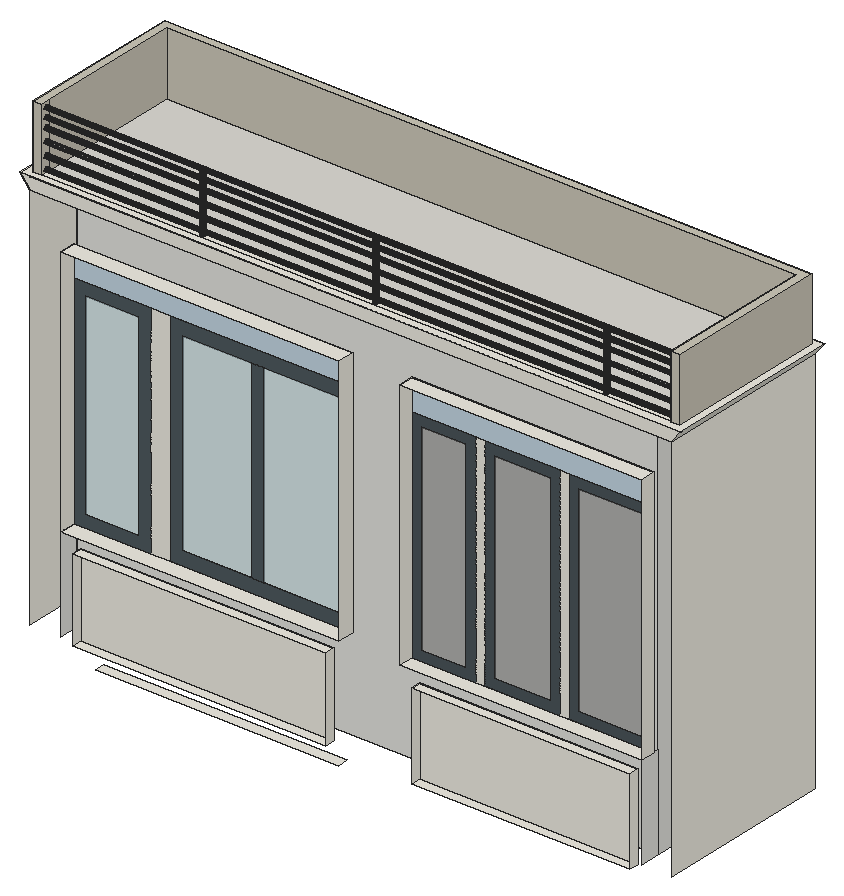
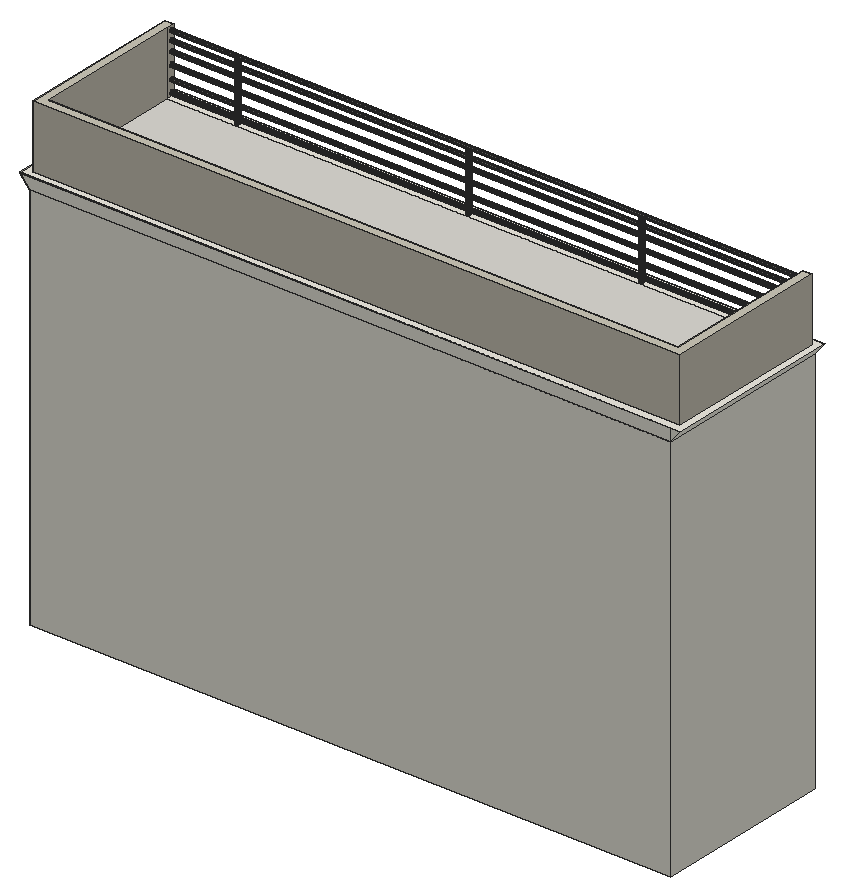
# SketchUp Ruby script. Lengths in inches.
U = 1.inch
M = Sketchup.active_model
def pt(a) = Geom::Point3d.new(a.map { |v| v * U })
def face(e, loops, mat)
  f = e.add_face(loops[0].map { |a| pt(a) })
  loops[1..].each { |l| e.add_face(l.map { |a| pt(a) }).erase! }
  f.material = f.back_material = mat if mat
  f
end
# faces: each face lists its corners as indices into pts; further lists are holes
def faces(e, pts, list, mat = nil) = list.each { |f| face(e, (f[0].is_a?(Array) ? f : [f]).map { |l| l.map { |i| pts[i] } }, mat) }
# xy, xz, yz: faces in a plane at the given z, y or x. An outline is a flat list of corners, or four numbers for a rectangle; further outlines are holes
def ring(l) = l.size == 4 ? [[l[0], l[1]], [l[2], l[1]], [l[2], l[3]], [l[0], l[3]]] : l.each_slice(2).to_a
def flat(e, list, mat, &to3) = list.each { |f| face(e, (f[0].is_a?(Array) ? f : [f]).map { |l| ring(l).map { |u, v| to3.(u, v) } }, mat) }
def xy(e, z, list, mat = nil) = flat(e, list, mat) { |x, y| [x, y, z] }
def xz(e, y, list, mat = nil) = flat(e, list, mat) { |x, z| [x, y, z] }
def yz(e, x, list, mat = nil) = flat(e, list, mat) { |y, z| [x, y, z] }
def lines(e, pts, list) = list.each { |a, b| e.add_line(pt(pts[a]), pt(pts[b])) }
# prism: a flat outline (further loops are holes) pulled along v
def prism(e, loops, v, mat = nil)
  f = face(e, loops, mat); d = Geom::Vector3d.new(v.map { |x| x * U })
  f.pushpull(f.normal.samedirection?(d) ? d.length : -d.length)
end
def box(e, o, s, mat = nil) = prism(e, [[o, [o[0] + s[0], o[1], o[2]], [o[0] + s[0], o[1] + s[1], o[2]], [o[0], o[1] + s[1], o[2]]]], [0, 0, s[2]], mat)
def at(x, y, z, deg = 0) = Geom::Transformation.translation(pt([x, y, z])) * Geom::Transformation.rotation(ORIGIN, Z_AXIS, deg.degrees)
def axes(o, x, y, z) = Geom::Transformation.new([*x, 0, *y, 0, *z, 0, *pt(o).to_a, 1])
def part(name) = M.definitions.add(name)
# library, detail: a bought-in or finely detailed component or shape, given as its bounding box
def library(name, o, s) = part(name).tap { |d| box(d.entities, o, s) }
def detail(e, o, s) = box(e.add_group.entities, o, s)
def put(e, d, t, mat = nil) = e.add_instance(d, t).tap { |i| i.material = mat if mat }
def group(e, t, mat = nil) = e.add_group.tap { |g| g.transformation = t; g.material = mat if mat }.entities
root = M.entities
M.materials.add("[Formica Graystone]").color = [204, 199, 184]
M.materials.add("[Formica Speckled Grey]1").color = [75, 84, 89]
M.materials.add("[Formica Speckled Grey]2").color = [79, 89, 94]
M.materials.add("[Granite Light Gray]").color = [149, 148, 144]
M.materials.add("[Terrazzo Light Blue]").color = [196, 214, 227]
M.materials.add("[Terrazzo Tile Light]").color = [219, 217, 210]
M.materials.add("[Tile Limestone Large]").color = [237, 234, 224]
M.materials.add("[Translucent Glass Gray]").color = [128, 128, 128]
M.materials["[Translucent Glass Gray]"].alpha = 0.5
M.materials.add("[Translucent Glass Safety]").color = [204, 235, 244]
M.materials["[Translucent Glass Safety]"].alpha = 0.5
xy(root,328.93,[[111.93,233.86,355.29,244.48]],"[Tile Limestone Large]")
xy(root,338.4,[[428.87,233.86,647.75,243.17]],"[Tile Limestone Large]")
xy(root,342.19,[[88.43,233.86,342.93,244.04]],"[Tile Limestone Large]")
xy(root,346.625,[[76.4,254.16,659.08,383.27]])
xy(root,424.46,[[428.87,233.86,647.75,243.17]],"[Tile Limestone Large]")
xy(root,425.32,[[88.43,233.86,342.93,244.04]],"[Tile Limestone Large]")
xy(root,440.5625,[[76.4,233.86,355.29,251.23],[416.36,233.86,659.08,249.23]],"[Tile Limestone Large]")
xy(root,692.2,[[76.4,233.86,355.29,251.23],[416.36,233.86,659.08,249.23]],"[Tile Limestone Large]")
xy(root,737,[[46.1875,233.86,46.1875,413.49,689.3,413.49,689.3,233.86,659.08,233.86,659.08,383.27,76.4,383.27,76.4,233.86],[76.4,233.86,659.08,254.16],[76.4,254.16,659.08,383.27],[76.4,254.16,659.08,383.27]])
xy(root,749.625,[[43.22,241.02,43.22,406.33,691.7,406.33,691.7,241.02,682.63,241.02,682.63,397.26,52.29,397.26,52.29,241.02],[209.95,243.3,209.34,243.38,208.76,243.62,208.27,244,207.9,244.49,207.66,245.0625,207.58,245.68,207.66,246.29,207.9,246.87,208.27,247.36,208.76,247.73,209.34,247.97,209.95,248.05,210.57,247.97,211.14,247.73,211.63,247.36,212.01,246.87,212.25,246.29,212.33,245.68,212.25,245.0625,212.01,244.49,211.63,244,211.14,243.62,210.57,243.38],[383.14,243.3,382.52,243.38,381.95,243.62,381.46,244,381.08,244.49,380.85,245.0625,380.76,245.68,380.85,246.29,381.08,246.87,381.46,247.36,381.95,247.73,382.52,247.97,383.14,248.05,383.75,247.97,384.33,247.73,384.82,247.36,385.2,246.87,385.43,246.29,385.51,245.68,385.43,245.0625,385.2,244.49,384.82,244,384.33,243.62,383.75,243.38],[614.64,243.3,614.02,243.38,613.45,243.62,612.96,244,612.58,244.49,612.35,245.0625,612.26,245.68,612.35,246.29,612.58,246.87,612.96,247.36,613.45,247.73,614.02,247.97,614.64,248.05,615.25,247.97,615.83,247.73,616.32,247.36,616.7,246.87,616.93,246.29,617.01,245.68,616.93,245.0625,616.7,244.49,616.32,244,615.83,243.62,615.25,243.38]])
xy(root,749.625,[[52.29,250.09,682.63,397.26]],"[Terrazzo Tile Light]")
xy(root,749.625,[[[36.0625,233.86,698.86,413.49],[43.22,241.02,691.7,406.33]],[[52.29,241.02,682.63,250.09],[614.64,243.3,614.02,243.38,613.45,243.62,612.96,244,612.58,244.49,612.35,245.0625,612.26,245.68,612.35,246.29,612.58,246.87,612.96,247.36,613.45,247.73,614.02,247.97,614.64,248.05,615.25,247.97,615.83,247.73,616.32,247.36,616.7,246.87,616.93,246.29,617.01,245.68,616.93,245.0625,616.7,244.49,616.32,244,615.83,243.62,615.25,243.38],[209.95,243.3,209.34,243.38,208.76,243.62,208.27,244,207.9,244.49,207.66,245.0625,207.58,245.68,207.66,246.29,207.9,246.87,208.27,247.36,208.76,247.73,209.34,247.97,209.95,248.05,210.57,247.97,211.14,247.73,211.63,247.36,212.01,246.87,212.25,246.29,212.33,245.68,212.25,245.0625,212.01,244.49,211.63,244,211.14,243.62,210.57,243.38],[383.14,243.3,382.52,243.38,381.95,243.62,381.46,244,381.08,244.49,380.85,245.0625,380.76,245.68,380.85,246.29,381.08,246.87,381.46,247.36,381.95,247.73,382.52,247.97,383.14,248.05,383.75,247.97,384.33,247.73,384.82,247.36,385.2,246.87,385.43,246.29,385.51,245.68,385.43,245.0625,385.2,244.49,384.82,244,384.33,243.62,383.75,243.38]]],"[Tile Limestone Large]")
xy(root,808.62,[[383.14,243.3,383.75,243.38,383.8,243.4,382.48,243.4,382.52,243.38],[382.48,243.4,383.8,243.4,384.33,243.62,384.82,244,385.2,244.49,385.43,245.0625,385.51,245.68,385.43,246.29,385.2,246.87,385.17,246.9,381.11,246.9,381.08,246.87,380.85,246.29,380.76,245.68,380.85,245.0625,381.08,244.49,381.46,244,381.95,243.62],[381.11,246.9,385.17,246.9,384.82,247.36,384.33,247.73,383.75,247.97,383.14,248.05,382.52,247.97,381.95,247.73,381.46,247.36]])
xy(root,809.09,[[209.95,243.3,210.23,243.34,209.67,243.34],[209.67,243.34,210.23,243.34,210.57,243.38,211.14,243.62,211.63,244,212.01,244.49,212.25,245.0625,212.33,245.68,212.25,246.29,212.01,246.87,211.93,246.97,207.97,246.97,207.9,246.87,207.66,246.29,207.58,245.68,207.66,245.0625,207.9,244.49,208.27,244,208.76,243.62,209.34,243.38],[207.97,246.97,211.93,246.97,211.63,247.36,211.14,247.73,210.57,247.97,209.95,248.05,209.34,247.97,208.76,247.73,208.27,247.36]])
xy(root,809.3125,[[614.64,243.3,615.25,243.38,615.83,243.62,616.32,244,616.7,244.49,616.93,245.0625,617.01,245.68,616.93,246.29,616.7,246.87,616.32,247.36,615.83,247.73,615.25,247.97,614.64,248.05,614.02,247.97,613.45,247.73,612.96,247.36,612.58,246.87,612.35,246.29,612.26,245.68,612.35,245.0625,612.58,244.49,612.96,244,613.45,243.62,614.02,243.38]])
xy(root,812.8125,[[43.22,241.02,52.29,241.02,52.29,397.26,682.63,397.26,682.63,241.02,691.7,241.02,691.7,406.33,43.22,406.33]],"[Formica Graystone]")
xz(root,233.86,[[46.1875,749.1875,698.86,749.625]])
xz(root,233.86,[[46.1875,737,689.3,737,698.86,749.1875,46.1875,749.1875,46.1875,749.625,36.0625,749.625]],"[Tile Limestone Large]")
xz(root,241.02,[[43.22,749.625,52.29,812.8125],[682.63,749.625,691.7,812.8125]],"[Formica Graystone]")
xz(root,243.17,[[428.87,338.4,647.75,424.46]],"[Tile Limestone Large]")
xz(root,244.04,[[88.43,342.19,342.93,425.32]],"[Tile Limestone Large]")
xz(root,249.23,[[[416.36,440.5625,480.46,661.07],[426.18,450.39,470.64,651.24]],[[489.4,440.5625,565.3,661.07],[499.22,450.39,555.48,651.24]],[[574.24,440.5625,659.08,661.07],[584.07,450.39,649.26,651.24]]],"[Formica Speckled Grey]1")
xz(root,249.23,[[416.36,661.07,659.08,692.2]],"[Terrazzo Light Blue]")
xz(root,249.23,[[480.46,440.5625,489.4,661.07],[565.3,440.5625,574.24,661.07]],"[Tile Limestone Large]")
xz(root,249.23,[[426.18,450.39,470.64,651.24],[499.22,450.39,555.48,651.24],[584.07,450.39,649.26,651.24]],"[Translucent Glass Gray]")
xz(root,251.23,[[[76.4,440.5625,153.38,661.07],[88.41,452.58,141.37,649.05]],[[172.06,440.5625,355.29,661.07],[185.5,454,341.85,647.625]],[254.47,454,266.69,647.625]],"[Formica Speckled Grey]2")
xz(root,251.23,[[76.4,661.07,355.29,692.2]],"[Terrazzo Light Blue]")
xz(root,251.23,[[153.38,440.5625,172.06,661.07]],"[Tile Limestone Large]")
xz(root,251.23,[[88.41,452.58,141.37,649.05],[185.5,454,254.47,647.625],[266.69,454,341.85,647.625]],"[Translucent Glass Safety]")
xz(root,254.16,[[76.4,346.625,659.08,737]])
xz(root,383.27,[[76.4,346.625,659.08,737]])
xz(root,397.26,[[52.29,749.625,682.63,812.8125]],"[Formica Graystone]")
xz(root,406.33,[[43.22,749.625,691.7,812.8125]],"[Formica Graystone]")
xz(root,413.49,[[46.1875,346.625,689.3,737],[46.1875,737,36.0625,749.625,698.86,749.625,698.86,749.1875,46.1875,749.1875],[46.1875,737,46.1875,749.1875,698.86,749.1875,689.3,737]],"[Tile Limestone Large]")
yz(root,43.22,[[241.02,749.625,406.33,812.8125]],"[Formica Graystone]")
yz(root,46.1875,[[233.86,346.625,413.49,737]],"[Tile Limestone Large]")
yz(root,52.29,[[245.15,751.4,244.68,751.46,244.25,751.65,243.87,751.93,243.58,752.31,243.4,752.75,243.34,753.22,243.4,753.68,243.58,754.12,243.87,754.5,244.25,754.78,244.68,754.97,245.15,755.03,245.62,754.97,246.06,754.78,246.43,754.5,246.72,754.12,246.9,753.68,246.97,753.22,246.9,752.75,246.72,752.31,246.43,751.93,246.06,751.65,245.62,751.46],[245.15,763.65,244.68,763.71,244.25,763.9,243.87,764.18,243.58,764.56,243.4,765,243.34,765.47,243.4,765.93,243.58,766.37,243.87,766.75,244.25,767.03,244.68,767.22,245.15,767.28,245.62,767.22,246.06,767.03,246.43,766.75,246.72,766.37,246.9,765.93,246.97,765.47,246.9,765,246.72,764.56,246.43,764.18,246.06,763.9,245.62,763.71],[245.15,776.34,244.68,776.4,244.25,776.58,243.87,776.87,243.58,777.25,243.4,777.68,243.34,778.15,243.4,778.62,243.58,779.06,243.87,779.43,244.25,779.72,244.68,779.9,245.15,779.97,245.62,779.9,246.06,779.72,246.43,779.43,246.72,779.06,246.9,778.62,246.97,778.15,246.9,777.68,246.72,777.25,246.43,776.87,246.06,776.58,245.62,776.4],[245.15,788.72,244.68,788.78,244.25,788.96,243.87,789.25,243.58,789.62,243.4,790.06,243.34,790.53,243.4,791,243.58,791.43,243.87,791.81,244.25,792.1,244.68,792.28,245.15,792.34,245.62,792.28,246.06,792.1,246.43,791.81,246.72,791.43,246.9,791,246.97,790.53,246.9,790.06,246.72,789.62,246.43,789.25,246.06,788.96,245.62,788.78],[245.15,798.28,244.68,798.34,244.25,798.52,243.87,798.81,243.58,799.18,243.4,799.62,243.34,800.09,243.4,800.56,243.58,801,243.87,801.37,244.25,801.66,244.68,801.84,245.15,801.9,245.62,801.84,246.06,801.66,246.43,801.37,246.72,801,246.9,800.56,246.97,800.09,246.9,799.62,246.72,799.18,246.43,798.81,246.06,798.52,245.62,798.34],
  [245.15,807.28,244.68,807.34,244.25,807.52,243.87,807.81,243.58,808.18,243.4,808.62,243.34,809.09,243.4,809.56,243.58,810,243.87,810.37,244.25,810.66,244.68,810.84,245.15,810.9,245.62,810.84,246.06,810.66,246.43,810.37,246.72,810,246.9,809.56,246.97,809.09,246.9,808.62,246.72,808.18,246.43,807.81,246.06,807.52,245.62,807.34]])
yz(root,52.29,[[[241.02,749.625,250.09,812.8125],[245.15,807.28,244.68,807.34,244.25,807.52,243.87,807.81,243.58,808.18,243.4,808.62,243.34,809.09,243.4,809.56,243.58,810,243.87,810.37,244.25,810.66,244.68,810.84,245.15,810.9,245.62,810.84,246.06,810.66,246.43,810.37,246.72,810,246.9,809.56,246.97,809.09,246.9,808.62,246.72,808.18,246.43,807.81,246.06,807.52,245.62,807.34],[245.15,751.4,244.68,751.46,244.25,751.65,243.87,751.93,243.58,752.31,243.4,752.75,243.34,753.22,243.4,753.68,243.58,754.12,243.87,754.5,244.25,754.78,244.68,754.97,245.15,755.03,245.62,754.97,246.06,754.78,246.43,754.5,246.72,754.12,246.9,753.68,246.97,753.22,246.9,752.75,246.72,752.31,246.43,751.93,246.06,751.65,245.62,751.46],[245.15,798.28,244.68,798.34,244.25,798.52,243.87,798.81,243.58,799.18,243.4,799.62,243.34,800.09,243.4,800.56,243.58,801,243.87,801.37,244.25,801.66,244.68,801.84,245.15,801.9,245.62,801.84,246.06,801.66,246.43,801.37,246.72,801,246.9,800.56,246.97,800.09,246.9,799.62,246.72,799.18,246.43,798.81,246.06,798.52,245.62,798.34],[245.15,763.65,244.68,763.71,244.25,763.9,243.87,764.18,243.58,764.56,243.4,765,243.34,765.47,243.4,765.93,243.58,766.37,243.87,766.75,244.25,767.03,244.68,767.22,245.15,767.28,245.62,767.22,246.06,767.03,246.43,766.75,246.72,766.37,246.9,765.93,246.97,765.47,246.9,765,246.72,764.56,246.43,764.18,246.06,763.9,245.62,763.71],[245.15,788.72,244.68,788.78,244.25,788.96,243.87,789.25,243.58,789.62,243.4,790.06,243.34,790.53,243.4,791,243.58,791.43,243.87,791.81,244.25,792.1,244.68,792.28,245.15,792.34,245.62,792.28,246.06,792.1,246.43,791.81,246.72,791.43,246.9,791,246.97,790.53,246.9,790.06,246.72,789.62,246.43,789.25,246.06,788.96,245.62,788.78],[245.15,776.34,244.68,776.4,244.25,776.58,243.87,776.87,243.58,777.25,243.4,777.68,243.34,778.15,243.4,778.62,243.58,779.06,243.87,779.43,244.25,779.72,244.68,779.9,245.15,779.97,245.62,779.9,246.06,779.72,246.43,779.43,246.72,779.06,246.9,778.62,246.97,778.15,246.9,777.68,246.72,777.25,246.43,776.87,246.06,776.58,245.62,776.4]],[250.09,749.625,397.26,812.8125]],"[Formica Graystone]")
yz(root,76.4,[[233.86,346.625,254.16,440.5625],[254.16,346.625,383.27,737]])
yz(root,76.4,[[233.86,440.5625,251.23,692.2]],"[Tile Limestone Large]")
yz(root,88.43,[[233.86,342.19,244.04,425.32]],"[Tile Limestone Large]")
yz(root,342.93,[[233.86,342.19,244.04,425.32]],"[Tile Limestone Large]")
yz(root,355.29,[[233.86,440.5625,251.23,692.2]],"[Tile Limestone Large]")
yz(root,416.36,[[233.86,440.5625,249.23,692.2]],"[Tile Limestone Large]")
yz(root,428.87,[[233.86,338.4,243.17,424.46]],"[Tile Limestone Large]")
yz(root,647.75,[[233.86,338.4,243.17,424.46]],"[Tile Limestone Large]")
yz(root,659.08,[[233.86,346.625,254.16,440.5625],[254.16,346.625,383.27,737]])
yz(root,659.08,[[233.86,440.5625,249.23,692.2]],"[Tile Limestone Large]")
yz(root,682.63,[[[241.02,749.625,250.09,812.8125],[245.15,807.28,245.62,807.34,246.06,807.52,246.43,807.81,246.72,808.18,246.9,808.62,246.97,809.09,246.9,809.56,246.72,810,246.43,810.37,246.06,810.66,245.62,810.84,245.15,810.9,244.68,810.84,244.25,810.66,243.87,810.37,243.58,810,243.4,809.56,243.34,809.09,243.4,808.62,243.58,808.18,243.87,807.81,244.25,807.52,244.68,807.34],[245.15,798.28,245.62,798.34,246.06,798.52,246.43,798.81,246.72,799.18,246.9,799.62,246.97,800.09,246.9,800.56,246.72,801,246.43,801.37,246.06,801.66,245.62,801.84,245.15,801.9,244.68,801.84,244.25,801.66,243.87,801.37,243.58,801,243.4,800.56,243.34,800.09,243.4,799.62,243.58,799.18,243.87,798.81,244.25,798.52,244.68,798.34],[245.15,788.72,245.62,788.78,246.06,788.96,246.43,789.25,246.72,789.62,246.9,790.06,246.97,790.53,246.9,791,246.72,791.43,246.43,791.81,246.06,792.1,245.62,792.28,245.15,792.34,244.68,792.28,244.25,792.1,243.87,791.81,243.58,791.43,243.4,791,243.34,790.53,243.4,790.06,243.58,789.62,243.87,789.25,244.25,788.96,244.68,788.78],[245.15,776.34,245.62,776.4,246.06,776.58,246.43,776.87,246.72,777.25,246.9,777.68,246.97,778.15,246.9,778.62,246.72,779.06,246.43,779.43,246.06,779.72,245.62,779.9,245.15,779.97,244.68,779.9,244.25,779.72,243.87,779.43,243.58,779.06,243.4,778.62,243.34,778.15,243.4,777.68,243.58,777.25,243.87,776.87,244.25,776.58,244.68,776.4],[245.15,751.4,245.62,751.46,246.06,751.65,246.43,751.93,246.72,752.31,246.9,752.75,246.97,753.22,246.9,753.68,246.72,754.12,246.43,754.5,246.06,754.78,245.62,754.97,245.15,755.03,244.68,754.97,244.25,754.78,243.87,754.5,243.58,754.12,243.4,753.68,243.34,753.22,243.4,752.75,243.58,752.31,243.87,751.93,244.25,751.65,244.68,751.46],[245.15,763.65,245.62,763.71,246.06,763.9,246.43,764.18,246.72,764.56,246.9,765,246.97,765.47,246.9,765.93,246.72,766.37,246.43,766.75,246.06,767.03,245.62,767.22,245.15,767.28,244.68,767.22,244.25,767.03,243.87,766.75,243.58,766.37,243.4,765.93,243.34,765.47,243.4,765,243.58,764.56,243.87,764.18,244.25,763.9,244.68,763.71]],[250.09,749.625,397.26,812.8125]],"[Formica Graystone]")
yz(root,689.3,[[233.86,346.625,413.49,737]],"[Tile Limestone Large]")
yz(root,691.7,[[241.02,749.625,406.33,812.8125]],"[Formica Graystone]")
yz(root,698.86,[[233.86,749.1875,413.49,749.625]])
p = [[46.1875,233.86,737],[36.0625,233.86,749.625],[36.0625,413.49,749.625],[46.1875,413.49,737],[698.86,233.86,749.1875],[689.3,233.86,737],
  [689.3,413.49,737],[698.86,413.49,749.1875],[209.34,243.38,749.625],[209.95,243.3,749.625],[209.95,243.3,809.09],[209.67,243.34,809.09],
  [209.34,243.38,809.09],[210.57,243.38,749.625],[210.57,243.38,809.09],[210.23,243.34,809.09],[382.52,243.38,749.625],[383.14,243.3,749.625],
  [383.14,243.3,808.62],[382.52,243.38,808.62],[383.75,243.38,749.625],[383.75,243.38,808.62],[614.02,243.38,749.625],[614.64,243.3,749.625],
  [614.64,243.3,809.3125],[614.02,243.38,809.3125],[615.25,243.38,749.625],[615.25,243.38,809.3125],[208.76,243.62,749.625],[208.76,243.62,809.09],
  [211.14,243.62,749.625],[211.14,243.62,809.09],[381.95,243.62,749.625],[382.48,243.4,808.62],[381.95,243.62,808.62],[384.33,243.62,749.625],
  [384.33,243.62,808.62],[383.8,243.4,808.62],[613.45,243.62,749.625],[613.45,243.62,809.3125],[615.83,243.62,749.625],[615.83,243.62,809.3125],
  [208.27,244,749.625],[208.27,244,809.09],[211.63,244,749.625],[211.63,244,809.09],[381.46,244,749.625],[381.46,244,808.62],
  [384.82,244,749.625],[384.82,244,808.62],[612.96,244,749.625],[612.96,244,809.3125],[616.32,244,749.625],[616.32,244,809.3125],
  [207.9,244.49,749.625],[207.9,244.49,809.09],[212.01,244.49,749.625],[212.01,244.49,809.09],[381.08,244.49,749.625],[381.08,244.49,808.62],
  [385.2,244.49,749.625],[385.2,244.49,808.62],[612.58,244.49,749.625],[612.58,244.49,809.3125],[616.7,244.49,749.625],[616.7,244.49,809.3125],
  [207.66,245.0625,749.625],[207.66,245.0625,809.09],[212.25,245.0625,749.625],[212.25,245.0625,809.09],[380.85,245.0625,749.625],[380.85,245.0625,808.62],
  [385.43,245.0625,749.625],[385.43,245.0625,808.62],[612.35,245.0625,749.625],[612.35,245.0625,809.3125],[616.93,245.0625,749.625],[616.93,245.0625,809.3125],
  [207.58,245.68,749.625],[207.58,245.68,809.09],[212.33,245.68,749.625],[212.33,245.68,809.09],[380.76,245.68,749.625],[380.76,245.68,808.62],
  [385.51,245.68,749.625],[385.51,245.68,808.62],[612.26,245.68,749.625],[612.26,245.68,809.3125],[617.01,245.68,749.625],[617.01,245.68,809.3125],
  [207.66,246.29,749.625],[207.66,246.29,809.09],[212.25,246.29,749.625],[212.25,246.29,809.09],[380.85,246.29,749.625],[380.85,246.29,808.62],
  [385.43,246.29,749.625],[385.43,246.29,808.62],[612.35,246.29,749.625],[612.35,246.29,809.3125],[616.93,246.29,749.625],[616.93,246.29,809.3125],
  [207.9,246.87,749.625],[207.9,246.87,809.09],[212.01,246.87,749.625],[212.01,246.87,809.09],[381.08,246.87,749.625],[381.08,246.87,808.62],
  [385.2,246.87,749.625],[385.2,246.87,808.62],[612.58,246.87,749.625],[612.58,246.87,809.3125],[616.7,246.87,749.625],[616.7,246.87,809.3125],
  [208.27,247.36,749.625],[207.97,246.97,809.09],[208.27,247.36,809.09],[211.63,247.36,749.625],[211.63,247.36,809.09],[211.93,246.97,809.09],
  [381.46,247.36,749.625],[381.11,246.9,808.62],[381.46,247.36,808.62],[384.82,247.36,749.625],[384.82,247.36,808.62],[385.17,246.9,808.62],
  [612.96,247.36,749.625],[612.96,247.36,809.3125],[616.32,247.36,749.625],[616.32,247.36,809.3125],[208.76,247.73,749.625],[208.76,247.73,809.09],
  [211.14,247.73,749.625],[211.14,247.73,809.09],[381.95,247.73,749.625],[381.95,247.73,808.62],[384.33,247.73,749.625],[384.33,247.73,808.62],
  [613.45,247.73,749.625],[613.45,247.73,809.3125],[615.83,247.73,749.625],[615.83,247.73,809.3125],[209.34,247.97,749.625],[209.34,247.97,809.09],
  [210.57,247.97,749.625],[210.57,247.97,809.09],[382.52,247.97,749.625],[382.52,247.97,808.62],[383.75,247.97,749.625],[383.75,247.97,808.62],
  [614.02,247.97,749.625],[614.02,247.97,809.3125],[615.25,247.97,749.625],[615.25,247.97,809.3125],[209.95,248.05,749.625],[209.95,248.05,809.09],
  [383.14,248.05,749.625],[383.14,248.05,808.62],[614.64,248.05,749.625],[614.64,248.05,809.3125],[52.29,244.68,751.46],[52.29,245.15,751.4],
  [682.63,245.15,751.4],[682.63,244.68,751.46],[52.29,245.62,751.46],[682.63,245.62,751.46],[52.29,244.25,751.65],[682.63,244.25,751.65],
  [52.29,246.06,751.65],[682.63,246.06,751.65],[52.29,243.87,751.93],[682.63,243.87,751.93],[52.29,246.43,751.93],[682.63,246.43,751.93],
  [52.29,243.58,752.31],[682.63,243.58,752.31],[52.29,246.72,752.31],[682.63,246.72,752.31],[52.29,243.4,752.75],[682.63,243.4,752.75],
  [52.29,246.9,752.75],[682.63,246.9,752.75],[52.29,243.34,753.22],[682.63,243.34,753.22],[52.29,246.97,753.22],[682.63,246.97,753.22],
  [52.29,243.4,753.68],[682.63,243.4,753.68],[52.29,246.9,753.68],[682.63,246.9,753.68],[52.29,243.58,754.12],[682.63,243.58,754.12],
  [52.29,246.72,754.12],[682.63,246.72,754.12],[52.29,243.87,754.5],[682.63,243.87,754.5],[52.29,246.43,754.5],[682.63,246.43,754.5],
  [52.29,244.25,754.78],[682.63,244.25,754.78],[52.29,246.06,754.78],[682.63,246.06,754.78],[52.29,244.68,754.97],[682.63,244.68,754.97],
  [52.29,245.62,754.97],[682.63,245.62,754.97],[52.29,245.15,755.03],[682.63,245.15,755.03],[52.29,244.25,763.9],[52.29,244.68,763.71],
  [682.63,244.68,763.71],[682.63,244.25,763.9],[52.29,245.15,763.65],[682.63,245.15,763.65],[52.29,245.62,763.71],[682.63,245.62,763.71],
  [52.29,246.06,763.9],[682.63,246.06,763.9],[52.29,243.87,764.18],[682.63,243.87,764.18],[52.29,246.43,764.18],[682.63,246.43,764.18],
  [52.29,243.58,764.56],[682.63,243.58,764.56],[52.29,246.72,764.56],[682.63,246.72,764.56],[52.29,243.4,765],[682.63,243.4,765],
  [52.29,246.9,765],[682.63,246.9,765],[52.29,243.34,765.47],[682.63,243.34,765.47],[52.29,246.97,765.47],[682.63,246.97,765.47],
  [52.29,243.4,765.93],[682.63,243.4,765.93],[52.29,246.9,765.93],[682.63,246.9,765.93],[52.29,243.58,766.37],[682.63,243.58,766.37],
  [52.29,246.72,766.37],[682.63,246.72,766.37],[52.29,243.87,766.75],[682.63,243.87,766.75],[52.29,246.43,766.75],[682.63,246.43,766.75],
  [52.29,244.25,767.03],[682.63,244.25,767.03],[52.29,246.06,767.03],[682.63,246.06,767.03],[52.29,244.68,767.22],[682.63,244.68,767.22],
  [52.29,245.62,767.22],[682.63,245.62,767.22],[52.29,245.15,767.28],[682.63,245.15,767.28],[52.29,244.68,776.4],[52.29,245.15,776.34],
  [682.63,245.15,776.34],[682.63,244.68,776.4],[52.29,245.62,776.4],[682.63,245.62,776.4],[52.29,244.25,776.58],[682.63,244.25,776.58],
  [52.29,246.06,776.58],[682.63,246.06,776.58],[52.29,243.87,776.87],[682.63,243.87,776.87],[52.29,246.43,776.87],[682.63,246.43,776.87],
  [52.29,243.58,777.25],[682.63,243.58,777.25],[52.29,246.72,777.25],[682.63,246.72,777.25],[52.29,243.4,777.68],[682.63,243.4,777.68],
  [52.29,246.9,777.68],[682.63,246.9,777.68],[52.29,243.34,778.15],[682.63,243.34,778.15],[52.29,246.97,778.15],[682.63,246.97,778.15],
  [52.29,243.4,778.62],[682.63,243.4,778.62],[52.29,246.9,778.62],[682.63,246.9,778.62],[52.29,243.58,779.06],[682.63,243.58,779.06],
  [52.29,246.72,779.06],[682.63,246.72,779.06],[52.29,243.87,779.43],[682.63,243.87,779.43],[52.29,246.43,779.43],[682.63,246.43,779.43],
  [52.29,244.25,779.72],[682.63,244.25,779.72],[52.29,246.06,779.72],[682.63,246.06,779.72],[52.29,244.68,779.9],[682.63,244.68,779.9],
  [52.29,245.62,779.9],[682.63,245.62,779.9],[52.29,245.15,779.97],[682.63,245.15,779.97],[52.29,244.68,788.78],[52.29,245.15,788.72],
  [682.63,245.15,788.72],[682.63,244.68,788.78],[52.29,245.62,788.78],[682.63,245.62,788.78],[52.29,244.25,788.96],[682.63,244.25,788.96],
  [52.29,246.06,788.96],[682.63,246.06,788.96],[52.29,243.87,789.25],[682.63,243.87,789.25],[52.29,246.43,789.25],[682.63,246.43,789.25],
  [52.29,243.58,789.62],[682.63,243.58,789.62],[52.29,246.72,789.62],[682.63,246.72,789.62],[52.29,243.4,790.06],[682.63,243.4,790.06],
  [52.29,246.9,790.06],[682.63,246.9,790.06],[52.29,243.34,790.53],[682.63,243.34,790.53],[52.29,246.97,790.53],[682.63,246.97,790.53],
  [52.29,243.4,791],[682.63,243.4,791],[52.29,246.9,791],[682.63,246.9,791],[52.29,243.58,791.43],[682.63,243.58,791.43],
  [52.29,246.72,791.43],[682.63,246.72,791.43],[52.29,243.87,791.81],[682.63,243.87,791.81],[52.29,246.43,791.81],[682.63,246.43,791.81],
  [52.29,244.25,792.1],[682.63,244.25,792.1],[52.29,246.06,792.1],[682.63,246.06,792.1],[52.29,244.68,792.28],[682.63,244.68,792.28],
  [52.29,245.62,792.28],[682.63,245.62,792.28],[52.29,245.15,792.34],[682.63,245.15,792.34],[52.29,244.25,798.52],[52.29,244.68,798.34],
  [682.63,244.68,798.34],[682.63,244.25,798.52],[52.29,245.15,798.28],[682.63,245.15,798.28],[52.29,245.62,798.34],[682.63,245.62,798.34],
  [52.29,246.06,798.52],[682.63,246.06,798.52],[52.29,243.87,798.81],[682.63,243.87,798.81],[52.29,246.43,798.81],[682.63,246.43,798.81],
  [52.29,243.58,799.18],[682.63,243.58,799.18],[52.29,246.72,799.18],[682.63,246.72,799.18],[52.29,243.4,799.62],[682.63,243.4,799.62],
  [52.29,246.9,799.62],[682.63,246.9,799.62],[52.29,243.34,800.09],[682.63,243.34,800.09],[52.29,246.97,800.09],[682.63,246.97,800.09],
  [52.29,243.4,800.56],[682.63,243.4,800.56],[52.29,246.9,800.56],[682.63,246.9,800.56],[52.29,243.58,801],[682.63,243.58,801],
  [52.29,246.72,801],[682.63,246.72,801],[52.29,243.87,801.37],[682.63,243.87,801.37],[52.29,246.43,801.37],[682.63,246.43,801.37],
  [52.29,244.25,801.66],[682.63,244.25,801.66],[52.29,246.06,801.66],[682.63,246.06,801.66],[52.29,244.68,801.84],[682.63,244.68,801.84],
  [52.29,245.62,801.84],[682.63,245.62,801.84],[52.29,245.15,801.9],[682.63,245.15,801.9],[52.29,244.25,807.52],[52.29,244.68,807.34],
  [682.63,244.68,807.34],[682.63,244.25,807.52],[52.29,245.15,807.28],[682.63,245.15,807.28],[52.29,245.62,807.34],[682.63,245.62,807.34],
  [52.29,246.06,807.52],[682.63,246.06,807.52],[52.29,243.87,807.81],[682.63,243.87,807.81],[52.29,246.43,807.81],[682.63,246.43,807.81],
  [52.29,243.58,808.18],[682.63,243.58,808.18],[52.29,246.72,808.18],[682.63,246.72,808.18],[52.29,243.4,808.62],[682.63,243.4,808.62],
  [52.29,246.9,808.62],[682.63,246.9,808.62],[52.29,243.34,809.09],[682.63,243.34,809.09],[52.29,246.97,809.09],[682.63,246.97,809.09],
  [52.29,243.4,809.56],[682.63,243.4,809.56],[52.29,246.9,809.56],[682.63,246.9,809.56],[52.29,243.58,810],[682.63,243.58,810],
  [52.29,246.72,810],[682.63,246.72,810],[52.29,243.87,810.37],[682.63,243.87,810.37],[52.29,246.43,810.37],[682.63,246.43,810.37],
  [52.29,244.25,810.66],[682.63,244.25,810.66],[52.29,246.06,810.66],[682.63,246.06,810.66],[52.29,244.68,810.84],[682.63,244.68,810.84],
  [52.29,245.62,810.84],[682.63,245.62,810.84],[52.29,245.15,810.9],[682.63,245.15,810.9]]
faces(root,p,[[0,1,2,3],[4,5,6,7]],"[Tile Limestone Large]")
faces(root,p,[[8,9,10,11,12],[9,13,14,15,10],[16,17,18,19],[17,20,21,18],[22,23,24,25],[23,26,27,24],[28,8,12,29],[13,30,31,14],
  [32,16,19,33,34],[20,35,36,37,21],[38,22,25,39],[26,40,41,27],[42,28,29,43],[30,44,45,31],[46,32,34,47],[35,48,49,36],
  [50,38,39,51],[40,52,53,41],[54,42,43,55],[44,56,57,45],[58,46,47,59],[48,60,61,49],[62,50,51,63],[52,64,65,53],
  [66,54,55,67],[56,68,69,57],[70,58,59,71],[60,72,73,61],[74,62,63,75],[64,76,77,65],[78,66,67,79],[68,80,81,69],
  [82,70,71,83],[72,84,85,73],[86,74,75,87],[76,88,89,77],[90,78,79,91],[80,92,93,81],[94,82,83,95],[84,96,97,85],
  [98,86,87,99],[88,100,101,89],[102,90,91,103],[92,104,105,93],[106,94,95,107],[96,108,109,97],[110,98,99,111],[100,112,113,101],
  [114,102,103,115,116],[104,117,118,119,105],[120,106,107,121,122],[108,123,124,125,109],[126,110,111,127],[112,128,129,113],[130,114,116,131],[117,132,133,118],
  [134,120,122,135],[123,136,137,124],[138,126,127,139],[128,140,141,129],[142,130,131,143],[132,144,145,133],[146,134,135,147],[136,148,149,137],
  [150,138,139,151],[140,152,153,141],[154,142,143,155],[144,154,155,145],[156,146,147,157],[148,156,157,149],[158,150,151,159],[152,158,159,153]],"[Formica Graystone]")
faces(root,p,[[160,161,162,163],[161,164,165,162],[166,160,163,167],[164,168,169,165],[170,166,167,171],[168,172,173,169],[174,170,171,175],[172,176,177,173],
  [178,174,175,179],[176,180,181,177],[182,178,179,183],[180,184,185,181],[186,182,183,187],[184,188,189,185],[190,186,187,191],[188,192,193,189],
  [194,190,191,195],[192,196,197,193],[198,194,195,199],[196,200,201,197],[202,198,199,203],[200,204,205,201],[206,202,203,207],[204,206,207,205],
  [208,209,210,211],[209,212,213,210],[212,214,215,213],[214,216,217,215],[218,208,211,219],[216,220,221,217],[222,218,219,223],[220,224,225,221],
  [226,222,223,227],[224,228,229,225],[230,226,227,231],[228,232,233,229],[234,230,231,235],[232,236,237,233],[238,234,235,239],[236,240,241,237],
  [242,238,239,243],[240,244,245,241],[246,242,243,247],[244,248,249,245],[250,246,247,251],[248,252,253,249],[254,250,251,255],[252,254,255,253],
  [256,257,258,259],[257,260,261,258],[262,256,259,263],[260,264,265,261],[266,262,263,267],[264,268,269,265],[270,266,267,271],[268,272,273,269],
  [274,270,271,275],[272,276,277,273],[278,274,275,279],[276,280,281,277],[282,278,279,283],[280,284,285,281],[286,282,283,287],[284,288,289,285],
  [290,286,287,291],[288,292,293,289],[294,290,291,295],[292,296,297,293],[298,294,295,299],[296,300,301,297],[302,298,299,303],[300,302,303,301],
  [304,305,306,307],[305,308,309,306],[310,304,307,311],[308,312,313,309],[314,310,311,315],[312,316,317,313],[318,314,315,319],[316,320,321,317],
  [322,318,319,323],[320,324,325,321],[326,322,323,327],[324,328,329,325],[330,326,327,331],[328,332,333,329],[334,330,331,335],[332,336,337,333],
  [338,334,335,339],[336,340,341,337],[342,338,339,343],[340,344,345,341],[346,342,343,347],[344,348,349,345],[350,346,347,351],[348,350,351,349],
  [352,353,354,355],[353,356,357,354],[356,358,359,357],[358,360,361,359],[362,352,355,363],[360,364,365,361],[366,362,363,367],[364,368,369,365],
  [370,366,367,371],[368,372,373,369],[374,370,371,375],[372,376,377,373],[378,374,375,379],[376,380,381,377],[382,378,379,383],[380,384,385,381],
  [386,382,383,387],[384,388,389,385],[390,386,387,391],[388,392,393,389],[394,390,391,395],[392,396,397,393],[398,394,395,399],[396,398,399,397],
  [400,401,402,403],[401,404,405,402],[404,406,407,405],[406,408,409,407],[410,400,403,411],[408,412,413,409],[414,410,411,415],[412,416,417,413],
  [418,414,415,419,37,33],[416,420,121,125,421,417],[422,418,33,37,419,423,15,11],[420,424,115,119,425,421,125,121],[426,422,11,15,423,427],[424,428,429,425,119,115],[430,426,427,431],[428,432,433,429],
  [434,430,431,435],[432,436,437,433],[438,434,435,439],[436,440,441,437],[442,438,439,443],[440,444,445,441],[446,442,443,447],[444,446,447,445]],"[Granite Light Gray]")
